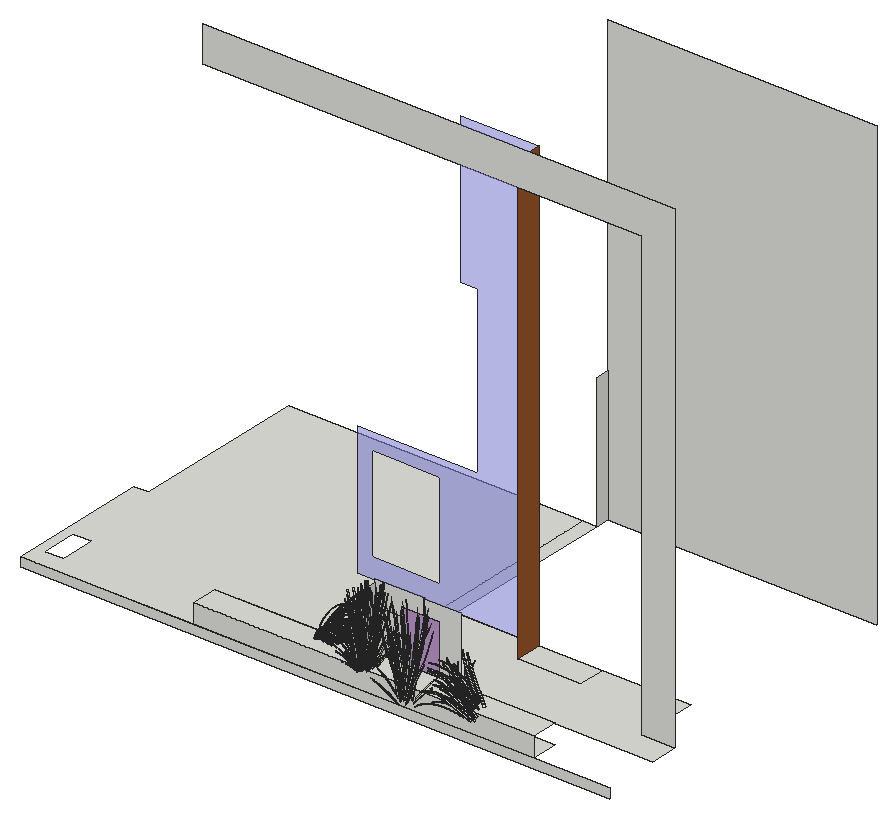
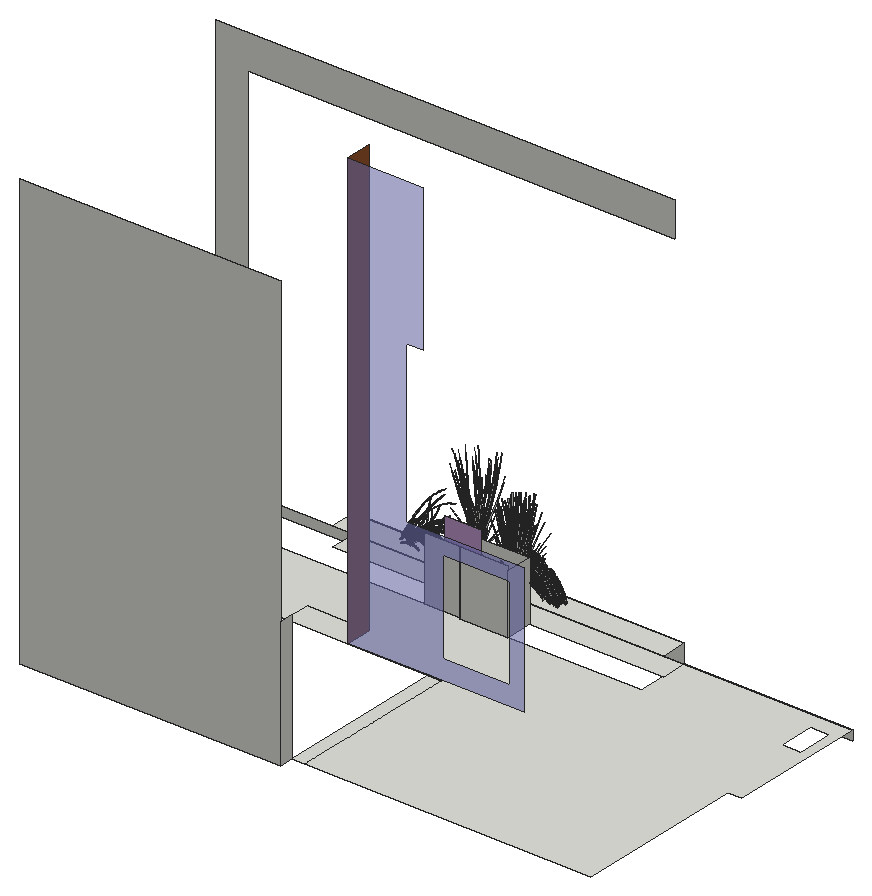
# SketchUp Ruby script. Lengths in inches.
U = 1.inch
M = Sketchup.active_model
def pt(a) = Geom::Point3d.new(a.map { |v| v * U })
def face(e, loops, mat)
  f = e.add_face(loops[0].map { |a| pt(a) })
  loops[1..].each { |l| e.add_face(l.map { |a| pt(a) }).erase! }
  f.material = f.back_material = mat if mat
  f
end
# faces: each face lists its corners as indices into pts; further lists are holes
def faces(e, pts, list, mat = nil) = list.each { |f| face(e, (f[0].is_a?(Array) ? f : [f]).map { |l| l.map { |i| pts[i] } }, mat) }
# xy, xz, yz: faces in a plane at the given z, y or x. An outline is a flat list of corners, or four numbers for a rectangle; further outlines are holes
def ring(l) = l.size == 4 ? [[l[0], l[1]], [l[2], l[1]], [l[2], l[3]], [l[0], l[3]]] : l.each_slice(2).to_a
def flat(e, list, mat, &to3) = list.each { |f| face(e, (f[0].is_a?(Array) ? f : [f]).map { |l| ring(l).map { |u, v| to3.(u, v) } }, mat) }
def xy(e, z, list, mat = nil) = flat(e, list, mat) { |x, y| [x, y, z] }
def xz(e, y, list, mat = nil) = flat(e, list, mat) { |x, z| [x, y, z] }
def yz(e, x, list, mat = nil) = flat(e, list, mat) { |y, z| [x, y, z] }
def lines(e, pts, list) = list.each { |a, b| e.add_line(pt(pts[a]), pt(pts[b])) }
# prism: a flat outline (further loops are holes) pulled along v
def prism(e, loops, v, mat = nil)
  f = face(e, loops, mat); d = Geom::Vector3d.new(v.map { |x| x * U })
  f.pushpull(f.normal.samedirection?(d) ? d.length : -d.length)
end
def box(e, o, s, mat = nil) = prism(e, [[o, [o[0] + s[0], o[1], o[2]], [o[0] + s[0], o[1] + s[1], o[2]], [o[0], o[1] + s[1], o[2]]]], [0, 0, s[2]], mat)
def at(x, y, z, deg = 0) = Geom::Transformation.translation(pt([x, y, z])) * Geom::Transformation.rotation(ORIGIN, Z_AXIS, deg.degrees)
def axes(o, x, y, z) = Geom::Transformation.new([*x, 0, *y, 0, *z, 0, *pt(o).to_a, 1])
def part(name) = M.definitions.add(name)
# library, detail: a bought-in or finely detailed component or shape, given as its bounding box
def library(name, o, s) = part(name).tap { |d| box(d.entities, o, s) }
def detail(e, o, s) = box(e.add_group.entities, o, s)
def put(e, d, t, mat = nil) = e.add_instance(d, t).tap { |i| i.material = mat if mat }
def group(e, t, mat = nil) = e.add_group.tap { |g| g.transformation = t; g.material = mat if mat }.entities
root = M.entities
M.materials.add("LightPink_Translucent").color = [144, 107, 117]
M.materials["LightPink_Translucent"].alpha = 0.75
M.materials.add("[Color I02]").color = [153, 153, 255]
M.materials["[Color I02]"].alpha = 0.56
M.materials.add("[Color L02]").color = [190, 153, 204]
M.materials.add("[Wood Cherry Original]").color = [152, 86, 42]
c1 = part("fur_instance\#8")
p = [[-0.25,1.49,0.03],[0.25,-1.49,-0.03],[0.44,-1.47,1.51],[-0.05,1.47,1.57],[0.65,-1.44,3.05],[0.16,1.45,3.11],
  [0.86,-1.42,4.59],[0.38,1.44,4.65],[1.1,-1.39,6.13],[0.62,1.43,6.18],[1.34,-1.35,7.66],[0.875,1.42,7.72],
  [1.6,-1.32,9.19],[1.14,1.41,9.25],[1.88,-1.28,10.72],[1.43,1.41,10.78],[2.18,-1.24,12.25],[1.73,1.41,12.3],
  [2.49,-1.19,13.77],[2.05,1.41,13.82],[2.83,-1.15,15.29],[2.4,1.41,15.34],[3.18,-1.09,16.8],[2.76,1.42,16.85],
  [3.56,-1.03,18.31],[3.14,1.43,18.35],[3.96,-0.97,19.81],[3.55,1.44,19.85],[4.38,-0.91,21.3],[3.99,1.46,21.35],
  [4.84,-0.83,22.78],[4.45,1.48,22.83],[5.32,-0.76,24.26],[4.93,1.51,24.31],[5.82,-0.67,25.73],[5.45,1.54,25.77],
  [6.36,-0.59,27.18],[6,1.57,27.23],[6.93,-0.49,28.625],[6.58,1.61,28.67],[7.54,-0.39,30.05],[7.19,1.66,30.1],
  [8.18,-0.28,31.47],[7.84,1.71,31.51],[8.85,-0.16,32.86],[8.53,1.77,32.9],[9.57,-0.04,34.24],[9.25,1.83,34.27],
  [10.32,0.09,35.59],[10.02,1.9,35.625],[11.12,0.23,36.92],[10.82,1.97,36.95],[11.95,0.38,38.22],[11.67,2.06,38.25],
  [12.84,0.54,39.49],[12.57,2.14,39.52],[13.76,0.71,40.73],[13.51,2.24,40.76],[14.73,0.89,41.93],[14.49,2.34,41.95],
  [15.75,1.08,43.09],[15.52,2.45,43.11],[16.82,1.28,44.2],[16.6,2.5625,44.23],[17.93,1.5,45.27],[17.73,2.68,45.29],
  [19.08,1.73,46.28],[18.9,2.81,46.3],[20.29,1.97,47.24],[20.125,2.93,47.26],[21.53,2.22,48.13],[21.39,3.0625,48.15],
  [22.82,2.5,48.96],[22.7,3.1875,48.98],[24.14,2.8125,49.72],[24.06,3.3,49.73],[25.48,3.27,50.41]]
faces(c1.entities,p,[[0,1,2,3],[3,2,4,5],[5,4,6,7],[7,6,8,9],[9,8,10,11],[11,10,12,13],[13,12,14,15],[15,14,16,17],
  [17,16,18,19],[19,18,20,21],[21,20,22,23],[23,22,24,25],[25,24,26,27],[27,26,28,29],[29,28,30,31],[31,30,32,33],
  [33,32,34,35],[35,34,36,37],[37,36,38,39],[39,38,40,41],[41,40,42,43],[43,42,44,45],[45,44,46,47],[47,46,48,49],
  [49,48,50,51],[51,50,52,53],[53,52,54,55],[55,54,56,57],[57,56,58,59],[59,58,60,61],[61,60,62,63],[63,62,64,65],
  [65,64,66,67],[67,66,68,69],[69,68,70,71],[71,70,72,73],[73,72,74,75],[75,74,76]])
c2 = part("blade")
p = [[2.15,0.21,22],[0,0.17,0],[0.09,0.45,0],[2.18,0.31,22],[2.29,0.31,22],[0.38,0.45,0],
  [2.48,0.24,33],[2.49,0.24,33],[2.48,0.22,33]]
faces(c2.entities,p,[[0,1,2,3],[4,5,2,3],[6,3,4,7],[8,0,3,6]])
c3 = part("blade with seeds\#1")
put(c3.entities,c2,at(0,0,0))
c4 = part("seeds")
p = [[0.3,-0.1,1.38],[-0.01,-0.03,1.59],[-0.01,-0.03,0.03],[0.14,-0.07,-0.07],[0.29,-0.03,3],[0.15,0.01,3.11]]
faces(c4.entities,p,[[0,1,2,3],[1,0,4,5]],"LightPink_Translucent")
c5 = part("blade with seeds")
put(c5.entities,c2,at(0,0,0))
put(c5.entities,c4,axes([2.4,0.25,30.99],[1.5799,-0.05474,1.17369],[-0.12525,1.92788,0.29478],[-0.07173,-0.02425,1.56792]))
xy(root,0,[[[1.2,32.99,110.38,32.99,110.38,67.24,228.64,67.24,228.64,66.43,373.22,66.43,373.22,84.18,352.27,84.18,352.27,122.8,296.76,122.8,296.76,105.55,256.63,105.55,256.63,122.8,195.57,122.8,195.57,233.8,10.2,233.8,10.2,122.8,1.2,122.8],[7.2,44,19.58,67.25]],[110.38,32.99,324.83,49.71],[256.63,105.55,296.76,122.8],[195.57,122.8,204.07,233.8]])
xy(root,12.375,[[110.38,32.99,324.83,49.71]])
xz(root,32.99,[[1.2,-6,373.22,0],[110.38,0,324.83,12.375]])
xz(root,49.71,[[197.22,0,228.64,12.375],[228.64,0,252.01,12.375],[197.22,12.375,228.64,38.5625]])
xz(root,49.71,[[228.64,12.375,252.01,43.9375]],"[Color L02]")
xz(root,66.43,[[228.64,0,252.01,41.375]])
xz(root,67.24,[[197.22,0,228.64,41.375]])
xz(root,84.18,[[352.27,0,373.22,0,373.22,304.31,75.43,304.31,75.43,282.04,352.27,282.04]])
xz(root,122.8,[[[142,0,256.63,0,256.63,282.04,207.32,282.04,207.32,187.31,218.2,187.31,218.2,84,142,84],[151.88,13.01,194.19,72.94]]],"[Color I02]")
xz(root,242.8,[[204.07,0,373.22,282.04]])
yz(root,197.22,[[49.71,0,49.71,38.5625,51.27,38.8125,67.24,38.8125,67.24,0]])
yz(root,204.07,[[233.8,0,242.8,84]])
yz(root,228.64,[[66.43,0,67.24,0,67.24,41.375,66.43,41.24]])
yz(root,256.63,[[105.55,0,122.8,282.04]],"[Wood Cherry Original]")
put(root,c1,axes([181.08,41.11,15.49],[0.28597,-0.0422,-0.27209],[0.30806,0.06306,0.085],[0.14113,-0.08271,0.33213]))
put(root,c1,axes([181.01,40.65,13.57],[0.35887,0.00033,-0.1558],[0.08324,0.0665,0.19531],[0.12369,-0.07249,0.29109]))
put(root,c1,axes([183.52,43.08,12.83],[-0.06872,-0.07861,0.22964],[0.27222,-0.04525,-0.15205],[0.23275,0.01718,0.23183]))
put(root,c1,axes([183.27,41.17,15.09],[0.02658,-0.086,-0.26556],[0.44346,0.03153,-0.16571],[0.20369,-0.08315,0.3671]))
put(root,c1,axes([186.21,44.29,13.78],[-0.33433,0.05756,0.18254],[-0.09078,-0.09599,0.28666],[0.2872,0.0212,0.28606]))
put(root,c1,axes([182.75,41.13,13.84],[0.12633,-0.0592,-0.22032],[0.30149,0.04949,-0.09622],[0.18794,-0.05619,0.28415]))
put(root,c1,axes([180.26,45.2,18.24],[0.47806,0.00311,-0.15218],[-0.07273,0.1252,-0.16437],[0.12473,0.01724,0.43913]))
put(root,c1,axes([184.64,44.99,13.39],[-0.06348,0.10676,-0.23569],[-0.37126,0.01698,0.24264],[0.24492,0.03533,0.28681]))
put(root,c1,axes([181.64,43.22,14.66],[0.32242,0.01145,-0.20079],[-0.10665,0.09325,-0.11686],[0.1669,0.01865,0.29249]))
put(root,c1,axes([180.69,40.59,14.02],[0.45116,-0.01744,-0.31391],[0.28883,0.06532,0.29637],[0.1442,-0.12309,0.33693]))
put(root,c1,axes([182.2,40.67,13.61],[0.23868,-0.03619,-0.37637],[0.38382,0.06071,0.06667],[0.19473,-0.10259,0.29985]))
put(root,c1,axes([183.59,42.65,13.69],[0.11192,-0.08912,0.00804],[0.27945,0.02654,-0.22763],[0.21064,-0.00191,0.28223]))
put(root,c1,axes([183.4,43.98,18],[0.18894,0.10942,-0.16061],[-0.40513,0.05851,0.15813],[0.20579,-0.01108,0.43033]))
put(root,c1,axes([183.53,42.08,14.17],[0.11489,-0.07964,-0.10676],[0.26936,0.04354,-0.20701],[0.22847,-0.02453,0.28315]))
put(root,c1,axes([184.78,42.125,13.18],[-0.05998,0.085,0.09028],[-0.2384,-0.03613,0.27279],[0.28483,-0.02324,0.23532]))
put(root,c1,axes([185.31,43.1875,13.43],[-0.13574,-0.08069,0.25732],[0.25291,-0.0632,-0.1678],[0.28624,0.00498,0.25641]))
put(root,c1,axes([181.625,46.91,14.18],[0.45812,0.00052,-0.21307],[-0.1395,0.10983,-0.31008],[0.14983,0.06381,0.32217]))
put(root,c1,axes([184.79,42.23,12.95],[-0.07354,-0.08857,0.14199],[0.23568,-0.02978,-0.24379],[0.27677,-0.00908,0.23332]))
put(root,c1,axes([185.68,44.94,14.36],[-0.13145,0.11602,-0.12661],[-0.33605,-0.01139,0.33056],[0.29915,0.02208,0.29796]))
put(root,c1,axes([185.59,41.63,13.74],[-0.12718,0.05977,0.28855],[-0.28671,-0.07195,0.16733],[0.2991,-0.05733,0.26791]))
put(root,c1,axes([182.28,44.71,13.71],[0.34239,-0.0692,0.00049],[0.16954,0.0685,-0.31793],[0.18221,0.04473,0.27113]))
put(root,c1,axes([186.05,41.63,13.55],[-0.15334,0.05521,0.30851],[-0.28262,-0.0784,0.14747],[0.30662,-0.05877,0.27465]))
put(root,c1,axes([182.79,42.63,14.42],[0.26324,-0.05399,-0.13586],[0.15137,0.0767,-0.18529],[0.21248,-0.00193,0.2847]))
put(root,c1,axes([183.23,41.44,14.08],[0.28294,0.0537,-0.13155],[-0.1326,0.06362,0.19986],[0.2113,-0.04676,0.2853]))
put(root,c1,axes([186.2,41.71,13.64],[-0.15346,-0.09619,-0.04526],[0.28391,-0.00341,-0.34021],[0.30776,-0.05899,0.27567]))
put(root,c1,axes([186.8125,42.68,13.15],[-0.21156,-0.07848,0.2314],[0.17827,-0.06816,-0.22589],[0.32055,-0.02616,0.26483]))
put(root,c1,axes([182.91,45.22,14.85],[0.43217,-0.01942,-0.15172],[-0.01396,0.11025,-0.23773],[0.15991,0.03296,0.35717]))
put(root,c1,axes([187.33,44.32,13.16],[-0.18837,0.10401,0.04187],[-0.26295,-0.05022,0.34364],[0.32256,0.00561,0.28895]))
put(root,c1,axes([184.94,41.2,13.98],[0.17538,0.08034,0.20651],[-0.37026,-0.00841,0.30749],[0.24651,-0.09013,0.29252]))
put(root,c1,axes([186.37,45.98,18.74],[0.149,0.13373,-0.19524],[-0.50514,0.05318,0.16911],[0.21416,-0.00071,0.49825]))
put(root,c1,axes([183.53,42.24,16.4],[0.38006,-0.02659,-0.21046],[0.13268,0.10254,-0.00753],[0.19596,-0.0403,0.38856]))
put(root,c1,axes([184,43.99,14.97],[0.28216,-0.08373,-0.05844],[0.24276,0.07079,-0.26184],[0.22513,0.01018,0.33528]))
put(root,c1,axes([184.48,42.39,13.18],[0.14514,-0.07667,-0.11085],[0.19944,0.05327,-0.25916],[0.27652,-0.00907,0.2331]))
put(root,c1,axes([183.42,43.48,15.57],[0.35003,-0.04511,-0.15955],[0.09912,0.09721,-0.20809],[0.22004,0.00995,0.32769]))
put(root,c1,axes([186.17,43.45,13.39],[0.01341,0.10477,-0.16669],[-0.30012,0.02304,0.27494],[0.29959,0.00521,0.26837]))
put(root,c1,axes([183.96,41.54,14.28],[0.3268,0.0025,-0.2446],[0.07821,0.08949,0.07984],[0.22723,-0.05028,0.30681]))
put(root,c1,axes([185.7,43.5,17.21],[0.24225,0.10443,-0.10996],[-0.37334,0.0621,0.20455],[0.2238,-0.03376,0.43344]))
put(root,c1,axes([184.57,41.88,14.875],[0.27807,-0.0377,-0.27012],[0.22134,0.08686,-0.03309],[0.24033,-0.05318,0.3245]))
put(root,c1,axes([189.26,43.72,13.07],[-0.26716,0.06653,0.25428],[-0.16996,-0.09969,0.25744],[0.35497,-0.01164,0.29924]))
put(root,c1,axes([184.28,41.42,14.5],[0.38112,0.01647,-0.22543],[0.04468,0.08907,0.16979],[0.22063,-0.06596,0.33357]))
put(root,c1,axes([190.13,41.73,13.12],[-0.36037,-0.10259,0.03375],[0.27114,-0.04204,-0.4404],[0.35172,-0.0931,0.35161]))
put(root,c1,axes([185.34,42.41,13.08],[0.1575,-0.07859,-0.12339],[0.20426,0.05791,-0.26768],[0.28915,-0.00948,0.24375]))
put(root,c1,axes([184.0625,42.4375,17.97],[0.48106,0.03048,-0.16267],[-0.07182,0.10935,0.18922],[0.18917,-0.06757,0.4507]))
put(root,c1,axes([185.26,44.32,16.37],[0.24181,0.08937,-0.26301],[-0.31272,0.08321,0.14244],[0.27661,-0.00251,0.37062]))
put(root,c1,axes([184.59,42.27,14.94],[0.31744,0.03739,-0.24659],[-0.09027,0.09521,0.09002],[0.25749,-0.02765,0.31911]))
put(root,c1,axes([185.42,41.91,13.51],[0.15887,-0.05533,-0.25915],[0.22278,0.07676,-0.17182],[0.29933,-0.03982,0.25215]))
put(root,c1,axes([184.32,41.27,15.71],[0.48158,-0.02516,-0.29827],[0.25745,0.09531,0.21951],[0.18335,-0.10745,0.43148]))
put(root,c1,axes([185.53,41.92,14.07],[0.2794,-0.03999,-0.25682],[0.19319,0.09103,-0.07563],[0.25448,-0.04072,0.32228]))
put(root,c1,axes([185.01,45.16,15.4375],[0.42563,0.00179,-0.2399],[-0.09167,0.12044,-0.17653],[0.21398,0.02392,0.37499]))
put(root,c1,axes([185.21,42.54,14.34],[0.32549,0.00157,-0.25975],[0.02664,0.10121,-0.00226],[0.2548,-0.02736,0.31578]))
put(root,c1,axes([187.91,44.49,13.29],[-0.00773,0.11759,-0.16367],[-0.3329,0.0176,0.31658],[0.33207,0.00578,0.29747]))
put(root,c1,axes([185.76,43.11,14.67],[0.26805,-0.06968,-0.17668],[0.22046,0.08432,-0.20691],[0.26458,-0.01545,0.334]))
put(root,c1,axes([187.7,42.01,13.15],[0.10291,0.0988,0.11051],[-0.31873,-0.01471,0.33861],[0.31939,-0.06122,0.28609]))
put(root,c1,axes([188.47,42.4375,13.29],[0.01573,0.10563,0.11224],[-0.31717,-0.03005,0.34297],[0.34739,-0.04621,0.29264]))
put(root,c1,axes([186.3,44.07,15.74],[0.34805,-0.06618,-0.18482],[0.1832,0.10189,-0.23326],[0.27522,-0.0025,0.36876]))
put(root,c1,axes([186.23,42.9,18.34],[0.47081,-0.0344,-0.26224],[0.19207,0.12202,0.03263],[0.22749,-0.06175,0.48221]))
put(root,c1,axes([193.69,43.78,13.84],[-0.35401,0.01108,0.43818],[-0.15381,-0.13302,0.01931],[0.42223,-0.05617,0.35568]))
put(root,c1,axes([189.1875,41.47,13.12],[0.2408,-0.04856,-0.44913],[0.43479,0.08513,-0.01404],[0.29905,-0.10934,0.35487]))
put(root,c1,axes([190.07,43.26,15.96],[0.11532,-0.11632,-0.19174],[0.42707,0.05687,-0.29119],[0.3314,-0.05303,0.4197]))
put(root,c1,axes([187.99,41.44,12.8125],[0.38774,0.0758,-0.1567],[-0.12803,0.06582,0.36795],[0.31846,-0.0843,0.31836]))
put(root,c1,axes([188.34,42.95,13.34],[0.29261,-0.0088,-0.34705],[0.06957,0.11266,-0.05611],[0.34848,-0.02844,0.28791]))
put(root,c1,axes([188.85,42.42,13.21],[0.32293,0.02966,-0.35036],[0.01889,0.10786,0.11122],[0.35386,-0.04707,0.29809]))
put(root,c1,axes([189.43,44.99,17.14],[0.29678,-0.10479,-0.1836],[0.33177,0.09329,-0.29677],[0.33935,-0.01982,0.42839]))
put(root,c1,axes([192.37,44.04,13.46],[0.16875,-0.10478,-0.22309],[0.30872,0.0806,-0.34547],[0.40765,-0.03327,0.33679]))
put(root,c3,axes([215.1875,32.05,14.1875],[0.15574,0.29248,1.11796],[-0.27258,0.87593,-0.24043],[-0.339,-0.16237,0.47799]))
put(root,c3,axes([214.89,36.58,14.1875],[0.2517,0.06231,1.11796],[0.2107,0.91089,-0.24043],[-0.32533,0.21292,0.47799]))
put(root,c3,axes([214.34,34.23,13.33],[0.02772,0.17259,1.37861],[-0.31204,0.95442,-0.21061],[-0.26028,-0.01601,0.23482]))
put(root,c3,axes([215.29,37.32,13.33],[0.10136,0.09967,1.37861],[0.21853,1.00724,-0.21061],[-0.1988,0.24333,0.23482]))
put(root,c3,axes([215.67,30.01,13.33],[-0.06061,0.15401,1.37861],[-0.67718,0.39559,-0.21061],[-0.18377,-0.26686,0.23482]))
put(root,c3,axes([218.08,35.65,13.8],[-0.789,0.42257,-0.54596],[-0.28415,-1.21723,-0.14329],[-0.26717,0.04671,1.20511]))
put(root,c3,axes([214.88,34.41,13.83],[0.4414,0.71104,-0.03043],[-0.48343,0.65151,-0.13798],[-0.13698,0.04587,0.45511]))
put(root,c3,axes([215.81,35.82,14.02],[-0.771,0.64332,0],[-0.42997,-1.07629,-0.40346],[-0.09793,-0.24513,1.27986]))
put(root,c3,axes([217.02,29.23,14.1875],[-0.02279,0.36758,1.11796],[-0.61135,0.37658,-0.24043],[-0.17294,-0.45158,0.47799]))
put(root,c3,axes([215.69,34.95,13.74],[-0.38471,-0.963,-0.38816],[0.68984,-0.5756,0],[-0.08762,-0.21933,1.23133]))
put(root,c3,axes([217.97,38.15,13.74],[-0.76941,0,-0.38816],[0,-1.1512,0],[-0.17524,0,1.23133]))
put(root,c3,axes([217.27,33.81,13.77],[-0.57832,-0.69306,-0.48746],[0.5244,-0.86095,-0.12794],[-0.14426,-0.27772,1.07599]))
put(root,c3,axes([215.68,37.94,13.83],[0.62826,0.29682,-0.03043],[-0.19326,0.91356,-0.13798],[-0.10276,0.13871,0.45511]))
put(root,c3,axes([218.28,35.01,13.89],[-0.6933,-0.49923,-0.34976],[0.33366,-1.03732,0.16833],[-0.15982,0,1.12298]))
put(root,c3,axes([217.9375,34.56,14.25],[-0.87795,0.1199,-0.22746],[-0.05308,-1.2488,-0.39091],[-0.11694,-0.2199,1.24856]))
put(root,c3,axes([217.99,37.65,13.75],[-0.48005,-0.71825,-0.24218],[0.48005,-0.71825,0.24218],[-0.15462,0,1.08647]))
put(root,c3,axes([218.86,35.14,14.25],[-0.36712,1.15878,-0.22746],[-0.77487,-0.55796,-0.39091],[-0.19025,0.03642,1.24856]))
put(root,c3,axes([218.55,38.43,14.02],[0,1.28663,0],[-0.85993,0,-0.40346],[-0.19586,0,1.27986]))
put(root,c3,axes([215.99,34.72,13.75],[0.19038,-0.95996,-0.24218],[0.67043,0.2417,0.24218],[-0.07731,-0.19353,1.08647]))
put(root,c3,axes([217.02,38.21,14.1875],[0.21421,-0.20089,1.11796],[0.58228,0.46292,-0.24043],[-0.13918,0.47533,0.47799]))
put(root,c3,axes([218.33,37.4375,13.98],[0.64687,0.95709,0.24045],[-0.64007,0.95767,-0.28529],[-0.1837,0.03342,1.28904]))
put(root,c3,axes([219.67,34.84,14.07],[-0.91172,-0.27272,-0.18316],[0.15892,-1.29308,0.40082],[-0.12591,0.22595,1.22302]))
put(root,c3,axes([218.68,37.65,14.1],[0.76941,0,0.38816],[0,1.1512,0],[-0.17524,0,1.23133]))
put(root,c3,axes([216,31.08,14.02],[-0.771,-0.64332,0],[0.42997,-1.07629,-0.40346],[0.09793,-0.24513,1.27986]))
put(root,c3,axes([218.39,34.81,14.01],[0.86036,-0.44736,0.3577],[0.29918,1.27824,0.14037],[-0.15809,-0.01562,1.24191]))
put(root,c3,axes([219.3,34.93,13.89],[-0.64581,0.61812,-0.34976],[-0.45477,-0.93627,0.16833],[-0.07991,0.20003,1.12298]))
put(root,c3,axes([219.05,28.55,13.71],[0.09234,0.66271,1.10687],[-0.73498,0.10548,0.06336],[-0.11125,-0.46416,0.62985]))
put(root,c3,axes([218.4,27.34,13.93],[-0.492,0.63792,-0.05072],[-0.45081,-0.69866,-0.22997],[-0.03174,-0.19797,0.75852]))
put(root,c3,axes([216.41,31.64,14.1],[-0.38471,0.963,0.38816],[-0.68984,-0.5756,0],[0.08762,-0.21933,1.23133]))
put(root,c3,axes([218.46,33.2,13.89],[-0.89027,0,0],[0,-1.28663,0],[0,0,1.40295]))
put(root,c3,axes([217.9,33.81,14.01],[0.69826,0.85315,0.3577],[-0.61637,1.01357,0.14037],[-0.06968,-0.20568,1.24191]))
put(root,c3,axes([219.55,35.49,13.77],[-0.12614,1.07035,-0.48746],[-0.77811,-0.22587,-0.12794],[-0.09429,0.31942,1.07599]))
put(root,c3,axes([217.37,35.74,13.41],[0.30804,1.01279,1.00794],[-0.88386,0.32236,0.39164],[0.0147,-0.62192,1.14642]))
put(root,c3,axes([219.15,32.875,13.96],[-0.66224,0.95709,-0.04793],[-0.66265,-0.95767,0],[-0.02313,0.03342,1.37258]))
put(root,c3,axes([217.6,33.02,14.21],[-0.68667,-0.1985,0.1132],[0.11919,-0.96981,-0.32325],[0.07051,-0.1765,0.99086]))
put(root,c3,axes([218.57,27.83,13.33],[-0.11681,0.05378,1.37861],[-0.6833,-0.37297,-0.21061],[-0.00983,-0.37623,0.23482]))
put(root,c3,axes([219.23,34.69,14.01],[0.16211,-1.30051,0.3577],[0.91555,0.26467,0.14037],[-0.08841,0.19006,1.24191]))
put(root,c3,axes([218.45,38.93,13.33],[0.12126,-0.02609,1.37861],[0.63324,0.52606,-0.21061],[-0.03192,0.37366,0.23482]))
put(root,c3,axes([220.74,36.625,13.75],[-0.67043,0.2417,-0.24218],[-0.19038,-0.95996,0.24218],[-0.07731,0.19353,1.08647]))
put(root,c3,axes([216.47,30.5,13.74],[0.38471,-0.963,-0.38816],[0.68984,0.5756,0],[0.08762,-0.21933,1.23133]))
put(root,c3,axes([217.83,33.12,14.25],[-0.51082,-1.03888,-0.22746],[0.72178,-0.69084,-0.39091],[0.0733,-0.25632,1.24856]))
put(root,c3,axes([219.67,34.28,14.25],[0.51082,1.03888,-0.22746],[-0.72178,0.69084,-0.39091],[-0.0733,0.25632,1.24856]))
put(root,c3,axes([221.02,36.89,13.74],[-0.38471,0.963,-0.38816],[-0.68984,-0.5756,0],[-0.08762,0.21933,1.23133]))
put(root,c3,axes([218.66,32.32,13.89],[0,-1.1512,0],[0.79656,0,0],[0,0,1.39475]))
put(root,c3,axes([216.76,30.76,13.75],[0.67043,-0.2417,-0.24218],[0.19038,0.95996,0.24218],[0.07731,-0.19353,1.08647]))
put(root,c3,axes([218.26,32.7,14.02],[-0.16211,1.30051,0.38462],[-0.91555,-0.26467,0.15093],[0.08841,-0.19006,1.33539]))
put(root,c3,axes([219.89,34.375,14.21],[0.68667,0.1985,0.1132],[-0.11919,0.96981,-0.32325],[-0.07051,0.1765,0.99086]))
put(root,c3,axes([220.52,33.73,13.88],[-0.66334,0.33572,0],[-0.2323,-0.95868,0],[0,0,1.20684]))
put(root,c3,axes([219,32.35,13.89],[0.49699,-0.71825,0],[0.49699,0.71825,0],[0,0,1.32329]))
put(root,c3,axes([220.42,32.48,13.87],[-0.26106,-1.08025,-0.15009],[0.75201,-0.37959,0.00006],[-0.02886,-0.11924,1.35949]))
put(root,c3,axes([217.94,31.9,13.77],[0.12614,-1.07035,-0.48746],[0.77811,0.22587,-0.12794],[0.09429,-0.31942,1.07599]))
put(root,c3,axes([219.9,33.11,14.09],[-0.61928,1.00474,-0.19695],[-0.6954,-0.84545,0.43099],[0.07244,0.27056,1.31508]))
put(root,c3,axes([220.82,33.97,13.88],[-0.34543,1.03732,0],[-0.71776,-0.49923,0],[0,0,1.27201]))
put(root,c3,axes([221.09,35.75,14.1],[0.38471,-0.963,0.38816],[0.68984,0.5756,0],[-0.08762,0.21933,1.23133]))
put(root,c3,axes([218.82,32.55,13.95],[0.88983,0,-0.04407],[0,1.28663,0],[0.02796,0,1.40226]))
put(root,c3,axes([218.1875,32.46,13.89],[0.64581,-0.61812,-0.34976],[0.45477,0.93627,0.16833],[0.07991,-0.20003,1.12298]))
put(root,c3,axes([221.49,36.31,14.02],[0.771,0.64332,0],[-0.42997,1.07629,-0.40346],[-0.09793,0.24513,1.27986]))
put(root,c3,axes([218.81,29.74,14.1],[-0.76941,0,0.38816],[0,-1.1512,0],[0.17524,0,1.23133]))
put(root,c3,axes([218.58,31.93,14.21],[-0.22438,-0.95868,0.1132],[0.64074,-0.33572,-0.32325],[0.14102,0,0.99086]))
put(root,c3,axes([219.77,33.62,13.89],[0.0475,1.11735,-0.34976],[-0.78843,0.10105,0.16833],[0.07991,0.20003,1.12298]))
put(root,c3,axes([220.14,28.36,14.1875],[-0.18923,0.24781,1.11796],[-0.626,-0.32242,-0.24043],[0.0848,-0.50137,0.47799]))
put(root,c3,axes([220.83,32.79,13.88],[0.34543,-1.03732,0],[0.71776,0.49923,0],[0,0,1.36775]))
put(root,c3,axes([219.72,32.6,14.21],[0.46228,-0.76018,0.1132],[0.52155,0.63409,-0.32325],[0.07051,0.1765,0.99086]))
put(root,c3,axes([221.6,32.38,13.875],[-0.77369,0.6353,-0.0402],[-0.42997,-1.07629,0.40346],[0.07366,0.26522,1.27923]))
put(root,c3,axes([220.54,33.17,13.95],[0.88392,-0.44736,-0.047],[0.30973,1.27824,0],[0.03087,-0.01562,1.34601]))
put(root,c3,axes([221.5,32.67,13.75],[-0.19038,0.95996,-0.24218],[-0.67043,-0.2417,0.24218],[0.07731,0.19353,1.08647]))
put(root,c3,axes([221.15,31.8,14.1],[-0.38471,-0.963,0.38816],[0.68984,-0.5756,0],[0.08762,0.21933,1.23133]))
put(root,c3,axes([219.38,29.47,13.88],[-0.00615,1.286,-0.0389],[-0.85993,0,0.39044],[0.19576,0.04041,1.23797]))
put(root,c3,axes([220.14,39.6,14.1875],[0.06316,-0.35759,1.11796],[0.64515,-0.23048,-0.24043],[0.12076,0.48573,0.47799]))
put(root,c3,axes([218.94,28.96,14.02],[0,-1.28663,0],[0.85993,0,-0.40346],[0.19586,0,1.27986]))
put(root,c3,axes([218.63,32.25,14.25],[0.36712,-1.15878,-0.22746],[0.77487,0.55796,-0.39091],[0.19025,-0.03642,1.24856]))
put(root,c3,axes([219.51,29.74,13.75],[0.48005,0.71825,-0.24218],[-0.48005,0.71825,0.24218],[0.15462,0,1.08647]))
put(root,c3,axes([219.55,32.83,14.25],[0.87795,-0.1199,-0.22746],[0.05308,1.2488,-0.39091],[0.11694,0.2199,1.24856]))
put(root,c3,axes([219.21,32.38,13.89],[0.6933,0.49923,-0.34976],[-0.33366,1.03732,0.16833],[0.15982,0,1.12298]))
put(root,c3,axes([220.22,33.59,13.77],[0.57832,0.69306,-0.48746],[-0.5244,0.86095,-0.12794],[0.14426,0.27772,1.07599]))
put(root,c3,axes([219.52,29.25,13.74],[0.76941,0,-0.38816],[0,1.1512,0],[0.17524,0,1.23133]))
put(root,c3,axes([221.8,32.44,13.74],[0.38471,0.963,-0.38816],[-0.68984,0.5756,0],[0.08762,0.21933,1.23133]))
put(root,c3,axes([221.2,32.35,13.98],[0.25008,-1.28817,0.24045],[0.8939,0.32227,-0.28529],[0.11188,0.21321,1.28904]))
put(root,c3,axes([219.42,31.79,13.8],[0.70446,-0.37729,-0.54108],[0.25371,1.08682,-0.14201],[0.23855,-0.0417,1.19435]))
put(root,c3,axes([221.68,31.57,14.02],[0.771,-0.64332,0],[0.42997,1.07629,-0.40346],[0.09793,0.24513,1.27986]))
put(root,c3,axes([221.94,30.54,13.33],[-0.11108,-0.07497,1.37861],[-0.32715,-0.94379,-0.21061],[0.16932,-0.28613,0.23482]))
put(root,c3,axes([221.85,39.21,13.33],[0.07687,-0.13802,1.37861],[0.71223,-0.23403,-0.21061],[0.15188,0.30589,0.23482]))
put(root,c3,axes([220.88,32.77,14.1875],[-0.25505,-0.01816,1.11796],[-0.28489,-0.86771,-0.24043],[0.30527,-0.26786,0.47799]))
put(root,c3,axes([221.92,34.95,13.33],[-0.04187,-0.16652,1.37861],[0.23044,-1.00168,-0.21061],[0.25972,-0.02929,0.23482]))
put(root,c3,axes([222.02,37.26,14.37],[-0.13625,-0.93474,0.05087],[0.54892,-0.21489,-0.67471],[0.27787,0.05926,0.60479]))
put(root,c3,axes([222.6,37.48,14.1875],[-0.12138,-0.3247,1.11796],[0.36598,-0.80168,-0.24043],[0.31668,0.23861,0.47799]))
put(root,c5,axes([249.87,19.47,13.89],[0.02447,0.14526,1.52927],[-0.4934,0.75861,-0.23362],[-0.35047,-0.03824,0.26049]))
put(root,c5,axes([249.61,23.54,13.89],[0.12945,0.09209,1.52927],[0.2195,0.85323,-0.23362],[-0.2869,0.18195,0.26049]))
put(root,c5,axes([253.1,20.78,14.38],[-1.0039,-0.15112,-0.54074],[0.21185,-0.93215,-0.14192],[-0.29959,-0.11295,1.19358]))
put(root,c5,axes([251.78,22.55,14.34],[-0.90321,-0.46087,-0.43058],[0.53987,-0.8264,0],[-0.20571,-0.10497,1.3659]))
put(root,c5,axes([251.39,15.68,13.89],[-0.09348,0.12142,1.52927],[-0.94472,0.26179,-0.23362],[-0.22822,-0.23815,0.26049]))
put(root,c5,axes([254.24,20.92,14.9],[-0.97439,0.61195,-0.25232],[-0.64795,-0.86467,-0.43363],[-0.24041,-0.08781,1.38501]))
put(root,c5,axes([252.03,22.2,14.35],[-0.2267,-0.80315,-0.26865],[0.90036,-0.22807,0.26865],[-0.18151,-0.09262,1.2052]))
put(root,c5,axes([254.89,21.59,14.38],[-0.65003,0.69281,-0.54074],[-0.8075,-0.62822,-0.14192],[-0.26048,0.17282,1.19358]))
put(root,c5,axes([255.33,21.2,14.73],[-0.94237,-0.74188,-0.21847],[0.79297,-0.83306,0.47809],[-0.25376,0.08678,1.45879]))
put(root,c5,axes([253.62,20.49,14.51],[-0.57975,-0.77365,-0.38798],[0.87815,-0.54479,0.18672],[-0.18761,-0.09573,1.2457]))
put(root,c5,axes([254.86,21.04,14.51],[-1.04798,0.0569,-0.38798],[-0.09477,-0.94451,0.18672],[-0.18761,0.09573,1.2457]))
put(root,c5,axes([253.71,20.93,14.71],[0.25579,-1.09221,-0.20318],[1.21281,0.19039,0.44463],[-0.21192,-0.15083,1.35668]))
put(root,c5,axes([255.96,23.48,14.34],[-0.90321,0.46087,-0.43058],[-0.53987,-0.8264,0],[-0.20571,0.10497,1.3659]))
put(root,c5,axes([250.61,18.89,14.34],[0,-0.92173,-0.43058],[1.07973,0,0],[0,-0.20993,1.3659]))
put(root,c5,axes([255.75,23.12,14.35],[-0.90036,-0.22807,-0.26865],[0.2267,-0.80315,0.26865],[-0.18151,0.09262,1.2052]))
put(root,c5,axes([253.43,19.96,14.9],[-1.08685,-0.4398,-0.25232],[0.52332,-0.92827,-0.43363],[-0.03416,-0.22791,1.38501]))
put(root,c5,axes([255.59,20.79,14.9],[0.11246,1.05175,-0.25232],[-1.17128,0.06359,-0.43363],[-0.20625,0.1401,1.38501]))
put(root,c5,axes([252.95,19.02,14.41],[-0.39633,-0.94519,-0.60562],[1.14167,-0.34041,-0.15895],[-0.04381,-0.32007,1.33681]))
put(root,c5,axes([251.07,18.91,14.35],[0.67366,-0.57509,-0.26865],[0.67366,0.57509,0.26865],[0,-0.18523,1.2052]))
put(root,c5,axes([254.28,14.54,13.89],[-0.16187,0.03321,1.52927],[-0.89517,-0.37382,-0.23362],[0.01502,-0.3118,0.26049]))
put(root,c5,axes([253.55,19.26,14.51],[0.46824,-0.83055,-0.38798],[0.97292,0.39972,0.18672],[0,-0.19146,1.2457]))
put(root,c5,axes([253.6,23.62,13.89],[0.15619,-0.05016,1.52927],[0.9395,0.27606,-0.23362],[0.02747,0.31114,0.26049]))
put(root,c5,axes([256.02,20.375,14.51],[-0.46824,0.83055,-0.38798],[-0.97292,-0.39972,0.18672],[0,0.19146,1.2457]))
put(root,c5,axes([258.49,20.73,14.35],[-0.67366,0.57509,-0.26865],[-0.67366,-0.57509,0.26865],[0,0.18523,1.2052]))
put(root,c5,axes([256.57,20.625,14.41],[0.35387,0.84392,-0.60022],[-1.01935,0.30394,-0.15753],[0.03911,0.28577,1.32487]))
put(root,c5,axes([253.98,18.85,14.9],[-0.11246,-1.05175,-0.25232],[1.17128,-0.06359,-0.43363],[0.20625,-0.1401,1.38501]))
put(root,c5,axes([256.13,19.6875,14.9],[1.08685,0.4398,-0.25232],[-0.52332,0.92827,-0.43363],[0.03416,0.22791,1.38501]))
put(root,c5,axes([253.82,16.52,14.35],[0.90036,0.22807,-0.26865],[-0.2267,0.80315,0.26865],[0.18151,-0.09262,1.2052]))
put(root,c5,axes([258.96,20.75,14.34],[0,0.92173,-0.43058],[-1.07973,0,0],[0,0.20993,1.3659]))
put(root,c5,axes([253.61,16.16,14.34],[0.90321,-0.46087,-0.43058],[0.53987,0.8264,0],[0.20571,-0.10497,1.3659]))
put(root,c5,axes([255.93,21.83,14.49],[1.01319,-0.31274,-0.16649],[0.35602,0.90088,0.00007],[0.11184,-0.03457,1.50806]))
put(root,c5,axes([255.95,19.15,14.51],[0.57975,0.77365,-0.38798],[-0.87815,0.54479,0.18672],[0.18761,0.09573,1.2457]))
put(root,c5,axes([254.68,18.05,14.38],[0.65003,-0.69281,-0.54074],[0.8075,0.62822,-0.14192],[0.26048,-0.17282,1.19358]))
put(root,c5,axes([257.53,17.4375,14.35],[0.2267,0.80315,-0.26865],[-0.90036,0.22807,0.26865],[0.18151,0.09262,1.2052]))
put(root,c5,axes([255.33,18.72,14.9],[0.97439,-0.61195,-0.25232],[0.64795,0.86467,-0.43363],[0.24041,0.08781,1.38501]))
put(root,c5,axes([252.87,18.17,13.97],[-0.94992,0.36903,1.11809],[-0.30235,-1.05883,0.43444],[0.58331,0.01761,1.2717]))
put(root,c5,axes([258.24,16.13,13.89],[-0.14445,-0.07261,1.52927],[-0.37103,-0.81124,-0.23362],[0.2503,-0.22015,0.26049]))
put(root,c5,axes([257.78,17.09,14.34],[0.90321,0.46087,-0.43058],[-0.53987,0.8264,0],[0.20571,0.10497,1.3659]))
put(root,c5,axes([257.74,23.65,13.89],[0.07031,-0.13307,1.52927],[0.8852,-0.39191,-0.23362],[0.26837,0.20284,0.26049]))
put(root,c5,axes([256.47,18.86,14.38],[1.0039,0.15112,-0.54074],[-0.21185,0.93215,-0.14192],[0.29959,0.11295,1.19358]))
put(root,c5,axes([260.29,19.61,13.89],[-0.05044,-0.13994,1.52927],[0.34982,-0.81857,-0.23362],[0.35288,-0.01177,0.26049]))
put(root,c1,axes([282.03,41.07,12.45],[-0.34304,-0.17032,-0.23502],[0.21672,-0.3457,0.25063],[-0.33871,0.00342,0.41909]))
put(root,c1,axes([283.48,37.27,13.11],[-0.16753,0.36241,-0.14436],[-0.34973,-0.08636,-0.30352],[-0.3374,-0.04095,0.40595]))
put(root,c1,axes([286.07,32.62,14.47],[-0.38475,0.24638,-0.22566],[-0.13971,-0.25484,-0.25837],[-0.3189,-0.13227,0.40665]))
put(root,c1,axes([284.74,35.58,13.24],[-0.24505,0.31939,-0.2117],[-0.28718,-0.17185,-0.24948],[-0.32846,-0.03987,0.3952]))
put(root,c1,axes([283.07,33.11,11.31],[-0.04449,-0.26129,-0.26766],[0.3381,-0.2268,0.30554],[-0.37513,-0.13013,0.32432]))
put(root,c1,axes([283.1875,30,9.44],[-0.16329,-0.12401,-0.41863],[0.39636,-0.27596,0.06589],[-0.3044,-0.23543,0.33316]))
put(root,c1,axes([284.5,37.04,11.76],[-0.18554,-0.28459,-0.08374],[0.321,-0.20739,0.30257],[-0.3095,0.00312,0.38294]))
put(root,c1,axes([286.86,36.22,10.4375],[-0.27599,-0.03055,-0.31164],[0.03613,-0.31664,0.15222],[-0.33797,0.02693,0.285]))
put(root,c1,axes([284.56,35.13,9.97],[0.03905,-0.3334,0.05525],[0.27854,-0.02716,0.3613],[-0.36347,-0.01992,0.2974]))
put(root,c1,axes([285.76,32.4,10.22],[-0.06673,-0.25395,-0.18532],[0.27318,-0.19572,0.30725],[-0.35059,-0.06777,0.28913]))
put(root,c1,axes([286.7,37.32,10.98],[-0.12388,0.27899,-0.30154],[-0.28541,-0.15849,-0.18902],[-0.32651,0.07205,0.29527]))
put(root,c1,axes([288.59,30.84,12.34],[-0.35295,0.12118,-0.26073],[0.00444,-0.28062,-0.13973],[-0.27499,-0.11406,0.35066]))
put(root,c1,axes([287.89,31.04,9.39],[-0.16318,0.27828,-0.12457],[-0.19465,-0.08021,-0.29921],[-0.31668,-0.06121,0.26116]))
put(root,c1,axes([288.71,30.86,15.09],[-0.48485,0.08322,-0.18647],[0.04075,-0.32102,-0.18484],[-0.19192,-0.18833,0.46761]))
put(root,c1,axes([285.8125,38.69,14.96],[-0.10281,0.37499,-0.10488],[-0.44091,-0.03463,-0.22679],[-0.25095,-0.02533,0.46823]))
put(root,c1,axes([288.3125,30.4375,10.1],[-0.22722,-0.00651,-0.32951],[0.15786,-0.28064,0.00614],[-0.30436,-0.10558,0.26313]))
put(root,c1,axes([289.51,28.47,10.12],[-0.27982,0.23702,-0.10525],[-0.12535,-0.11456,-0.31575],[-0.27827,-0.14781,0.26354]))
put(root,c1,axes([288.49,36.5625,11.17],[-0.25072,-0.20994,-0.08683],[0.2364,-0.23113,0.26489],[-0.25941,0.0376,0.34331]))
put(root,c1,axes([289.53,34.75,9.5625],[-0.26533,0.02068,-0.28176],[-0.0487,-0.27743,0.12578],[-0.28309,0.06247,0.256]))
put(root,c1,axes([284.81,34.39,10.31],[0.27564,-0.00662,0.35726],[-0.0561,0.33448,-0.07736],[-0.36351,-0.01992,0.29743]))
put(root,c1,axes([288.5,39.72,13.22],[-0.20486,0.28647,-0.29247],[-0.347,-0.18418,-0.09542],[-0.25833,0.07626,0.38236]))
put(root,c1,axes([284.5625,36.18,10.23],[0.28956,-0.07106,0.36279],[0.05237,0.32869,-0.05307],[-0.35729,0.02847,0.30129]))
put(root,c1,axes([285.77,37.42,12.28],[0.12337,0.31358,0.02766],[-0.34511,0.15109,-0.30909],[-0.30593,0.00309,0.37853]))
put(root,c1,axes([287.82,39.33,15.26],[-0.1624,0.35691,-0.17328],[-0.42297,-0.10144,-0.17105],[-0.23182,0.00564,0.46153]))
put(root,c1,axes([289.85,40,9.8125],[-0.30171,0.10787,-0.31065],[-0.20487,-0.26445,0.14302],[-0.23979,0.1404,0.28862]))
put(root,c1,axes([290.32,29.61,11.32],[-0.30859,0.16711,-0.19662],[-0.07348,-0.21803,-0.17893],[-0.24713,-0.10251,0.31514]))
put(root,c1,axes([290.3,31.85,11.2],[-0.28709,0.11718,-0.24868],[-0.06275,-0.25686,-0.05507],[-0.25569,-0.03103,0.30763]))
put(root,c1,axes([290.37,29.87,9.875],[-0.23084,0.11561,-0.27782],[-0.00863,-0.23665,-0.09845],[-0.288,-0.05567,0.23751]))
put(root,c1,axes([288.4375,35.46,17.4],[-0.34421,-0.22917,-0.13818],[0.37616,-0.30184,0.08888],[-0.16796,-0.09793,0.52531]))
put(root,c1,axes([290.05,35.88,10.45],[-0.25891,-0.18999,-0.05317],[0.16536,-0.20141,0.3129],[-0.26193,0.09996,0.26571]))
put(root,c1,axes([285.54,40.1,10.09],[0.31602,0.10859,0.2515],[-0.07193,0.3161,-0.27234],[-0.34011,0.07505,0.30757]))
put(root,c1,axes([285.42,36.96,11.3],[0.22552,-0.28523,0.24401],[0.27808,0.18514,0.1799],[-0.29887,0.00302,0.36979]))
put(root,c1,axes([287.46,33.75,10.71],[0.14434,-0.28883,0.19106],[0.21652,0.11117,0.27901],[-0.33628,-0.01843,0.27515]))
put(root,c1,axes([288.29,33.4,14.88],[-0.08498,-0.313,-0.10362],[0.41952,-0.14997,0.21784],[-0.24047,-0.0877,0.44182]))
